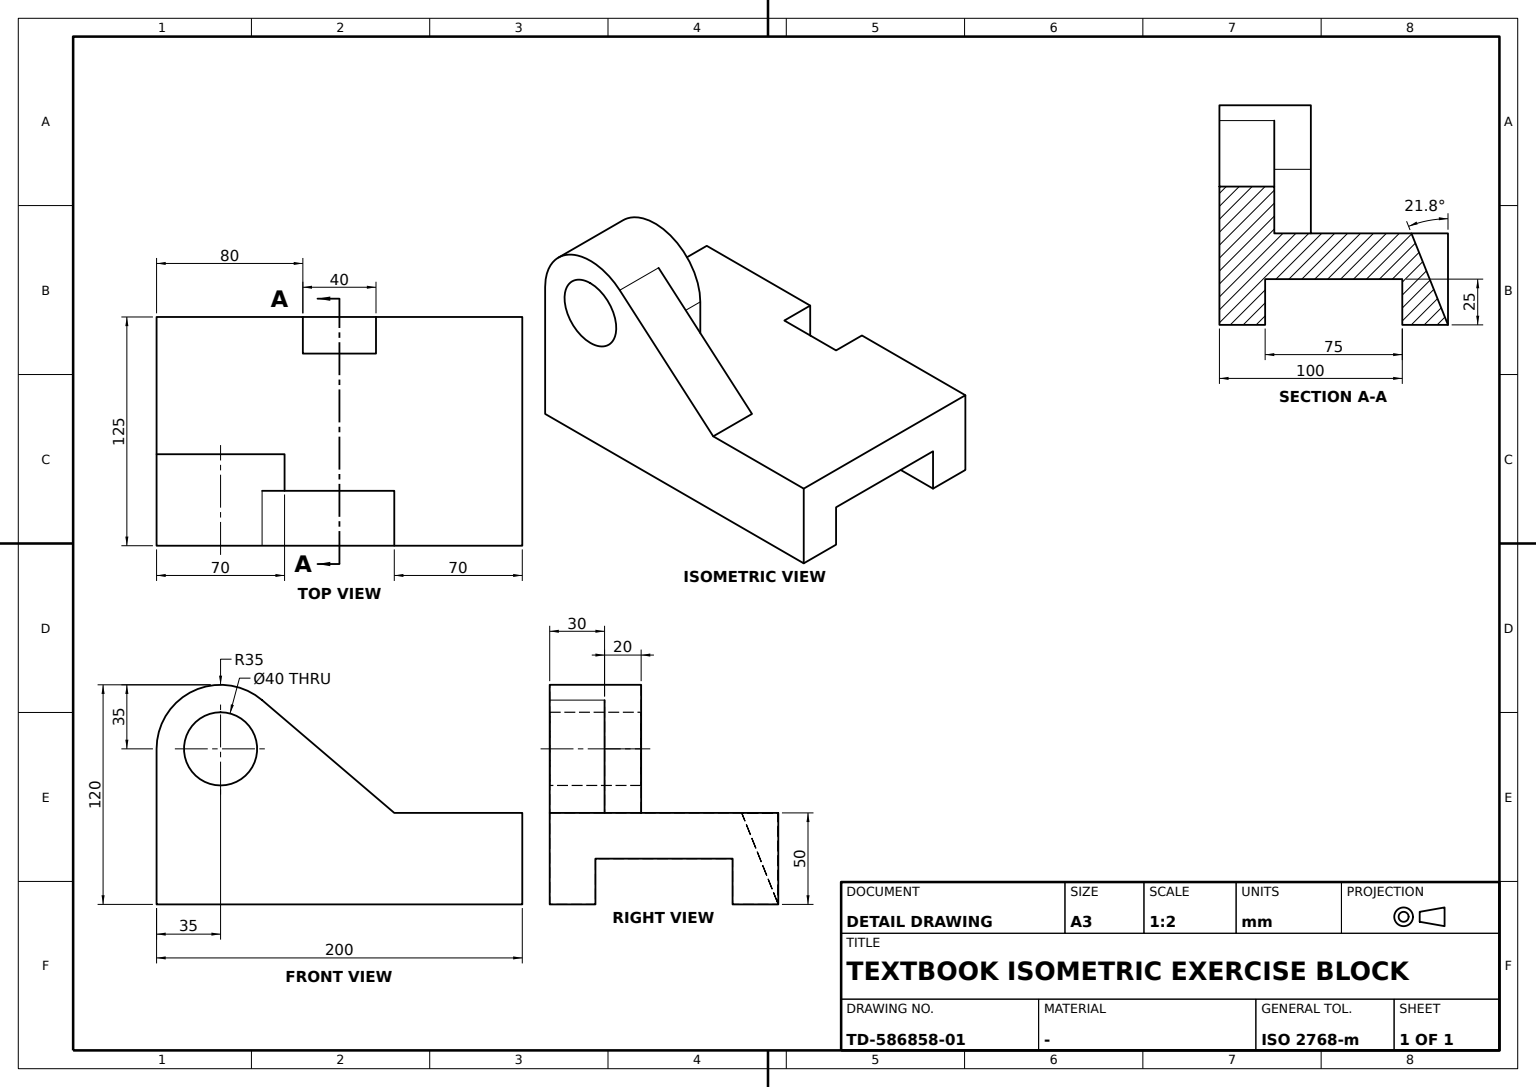
ISO-10303-21;
HEADER;
FILE_DESCRIPTION((''),'2;1');
FILE_NAME('','',(''),(''),'','','');
FILE_SCHEMA(('AUTOMOTIVE_DESIGN'));
ENDSEC;
DATA;
#1=APPLICATION_CONTEXT('');
#2=PRODUCT_CONTEXT('',#1,'mechanical');
#3=PRODUCT('','','',(#2));
#4=PRODUCT_DEFINITION_FORMATION('','',#3);
#5=PRODUCT_DEFINITION_CONTEXT('',#1,'design');
#6=PRODUCT_DEFINITION('','',#4,#5);
#7=PRODUCT_DEFINITION_SHAPE('','',#6);
#8=(LENGTH_UNIT()NAMED_UNIT(*)SI_UNIT(.MILLI.,.METRE.));
#9=(NAMED_UNIT(*)PLANE_ANGLE_UNIT()SI_UNIT($,.RADIAN.));
#10=(NAMED_UNIT(*)SI_UNIT($,.STERADIAN.)SOLID_ANGLE_UNIT());
#11=UNCERTAINTY_MEASURE_WITH_UNIT(LENGTH_MEASURE(0.005),#8,'distance_accuracy_value','');
#12=(GEOMETRIC_REPRESENTATION_CONTEXT(3)GLOBAL_UNCERTAINTY_ASSIGNED_CONTEXT((#11))GLOBAL_UNIT_ASSIGNED_CONTEXT((#8,#9,#10))REPRESENTATION_CONTEXT('',''));
#13=CARTESIAN_POINT('',(-20.,42.5,50.));
#14=VERTEX_POINT('',#13);
#15=CARTESIAN_POINT('',(-20.,62.5,0.));
#16=VERTEX_POINT('',#15);
#17=DIRECTION('',(0.,0.371390676,-0.928476691));
#18=VECTOR('',#17,1000.);
#19=LINE('',#13,#18);
#20=EDGE_CURVE('',#14,#16,#19,.T.);
#21=ORIENTED_EDGE('',*,*,#20,.T.);
#22=CARTESIAN_POINT('',(-20.,62.5,50.));
#23=VERTEX_POINT('',#22);
#24=DIRECTION('',(0.,0.,1.));
#25=VECTOR('',#24,1000.);
#26=LINE('',#22,#25);
#27=EDGE_CURVE('',#16,#23,#26,.T.);
#28=ORIENTED_EDGE('',*,*,#27,.T.);
#29=CARTESIAN_POINT('',(-20.,-62.5,50.));
#30=DIRECTION('',(0.,-1.,0.));
#31=VECTOR('',#30,1000.);
#32=LINE('',#29,#31);
#33=EDGE_CURVE('',#23,#14,#32,.T.);
#34=ORIENTED_EDGE('',*,*,#33,.T.);
#35=EDGE_LOOP('',(#21,#28,#34));
#36=FACE_BOUND('',#35,.T.);
#37=CARTESIAN_POINT('',(-20.,0.,0.));
#38=DIRECTION('',(1.,0.,0.));
#39=DIRECTION('',(0.,1.,0.));
#40=AXIS2_PLACEMENT_3D('',#37,#38,#39);
#41=PLANE('',#40);
#42=ADVANCED_FACE('',(#36),#41,.T.);
#43=CARTESIAN_POINT('',(-65.,-12.5,65.));
#44=VERTEX_POINT('',#43);
#45=CARTESIAN_POINT('',(-65.,-12.5,85.));
#46=DIRECTION('',(0.,0.,-1.));
#47=AXIS2_PLACEMENT_3D('',#45,#30,#46);
#48=CIRCLE('',#47,20.);
#49=EDGE_CURVE('',#44,#44,#48,.T.);
#50=ORIENTED_EDGE('',*,*,#49,.F.);
#51=EDGE_LOOP('',(#50));
#52=FACE_BOUND('',#51,.T.);
#53=CARTESIAN_POINT('',(-65.,-62.5,105.));
#54=VERTEX_POINT('',#53);
#55=CARTESIAN_POINT('',(-65.,-62.5,85.));
#56=AXIS2_PLACEMENT_3D('',#55,#39,#24);
#57=CIRCLE('',#56,20.);
#58=EDGE_CURVE('',#54,#54,#57,.F.);
#59=ORIENTED_EDGE('',*,*,#58,.T.);
#60=EDGE_LOOP('',(#59));
#61=FACE_BOUND('',#60,.T.);
#62=CARTESIAN_POINT('',(-65.,-37.5,85.));
#63=AXIS2_PLACEMENT_3D('',#62,#30,#38);
#64=CYLINDRICAL_SURFACE('',#63,20.);
#65=ADVANCED_FACE('',(#52,#61),#64,.F.);
#66=CARTESIAN_POINT('',(20.,62.5,50.));
#67=VERTEX_POINT('',#66);
#68=CARTESIAN_POINT('',(20.,42.5,50.));
#69=VERTEX_POINT('',#68);
#70=CARTESIAN_POINT('',(20.,-62.5,50.));
#71=LINE('',#70,#31);
#72=EDGE_CURVE('',#67,#69,#71,.T.);
#73=ORIENTED_EDGE('',*,*,#72,.F.);
#74=CARTESIAN_POINT('',(20.,62.5,0.));
#75=VERTEX_POINT('',#74);
#76=LINE('',#66,#25);
#77=EDGE_CURVE('',#75,#67,#76,.T.);
#78=ORIENTED_EDGE('',*,*,#77,.F.);
#79=LINE('',#68,#18);
#80=EDGE_CURVE('',#69,#75,#79,.T.);
#81=ORIENTED_EDGE('',*,*,#80,.F.);
#82=EDGE_LOOP('',(#73,#78,#81));
#83=FACE_BOUND('',#82,.T.);
#84=CARTESIAN_POINT('',(20.,0.,0.));
#85=AXIS2_PLACEMENT_3D('',#84,#38,#39);
#86=PLANE('',#85);
#87=ADVANCED_FACE('',(#83),#86,.F.);
#88=CARTESIAN_POINT('',(100.,-37.5,25.));
#89=VERTEX_POINT('',#88);
#90=CARTESIAN_POINT('',(100.,-37.5,0.));
#91=VERTEX_POINT('',#90);
#92=VECTOR('',#46,1000.);
#93=LINE('',#90,#92);
#94=EDGE_CURVE('',#89,#91,#93,.T.);
#95=ORIENTED_EDGE('',*,*,#94,.F.);
#96=CARTESIAN_POINT('',(100.,37.5,25.));
#97=VERTEX_POINT('',#96);
#98=CARTESIAN_POINT('',(100.,0.,25.));
#99=LINE('',#98,#31);
#100=EDGE_CURVE('',#97,#89,#99,.T.);
#101=ORIENTED_EDGE('',*,*,#100,.F.);
#102=CARTESIAN_POINT('',(100.,37.5,0.));
#103=VERTEX_POINT('',#102);
#104=LINE('',#102,#25);
#105=EDGE_CURVE('',#103,#97,#104,.T.);
#106=ORIENTED_EDGE('',*,*,#105,.F.);
#107=CARTESIAN_POINT('',(100.,62.5,0.));
#108=VERTEX_POINT('',#107);
#109=CARTESIAN_POINT('',(100.,0.,0.));
#110=LINE('',#109,#31);
#111=EDGE_CURVE('',#108,#103,#110,.T.);
#112=ORIENTED_EDGE('',*,*,#111,.F.);
#113=CARTESIAN_POINT('',(100.,62.5,50.));
#114=VERTEX_POINT('',#113);
#115=LINE('',#107,#92);
#116=EDGE_CURVE('',#114,#108,#115,.T.);
#117=ORIENTED_EDGE('',*,*,#116,.F.);
#118=CARTESIAN_POINT('',(100.,-62.5,50.));
#119=VERTEX_POINT('',#118);
#120=CARTESIAN_POINT('',(100.,0.,50.));
#121=VECTOR('',#39,1000.);
#122=LINE('',#120,#121);
#123=EDGE_CURVE('',#119,#114,#122,.T.);
#124=ORIENTED_EDGE('',*,*,#123,.F.);
#125=CARTESIAN_POINT('',(100.,-62.5,0.));
#126=VERTEX_POINT('',#125);
#127=LINE('',#125,#25);
#128=EDGE_CURVE('',#126,#119,#127,.T.);
#129=ORIENTED_EDGE('',*,*,#128,.F.);
#130=EDGE_CURVE('',#91,#126,#110,.T.);
#131=ORIENTED_EDGE('',*,*,#130,.F.);
#132=EDGE_LOOP('',(#95,#101,#106,#112,#117,#124,#129,#131));
#133=FACE_BOUND('',#132,.T.);
#134=AXIS2_PLACEMENT_3D('',#109,#38,#39);
#135=PLANE('',#134);
#136=ADVANCED_FACE('',(#133),#135,.T.);
#137=CARTESIAN_POINT('',(-100.,-12.5,50.));
#138=VERTEX_POINT('',#137);
#139=CARTESIAN_POINT('',(-30.,-12.5,50.));
#140=VERTEX_POINT('',#139);
#141=CARTESIAN_POINT('',(0.,-12.5,50.));
#142=VECTOR('',#38,1000.);
#143=LINE('',#141,#142);
#144=EDGE_CURVE('',#138,#140,#143,.T.);
#145=ORIENTED_EDGE('',*,*,#144,.F.);
#146=CARTESIAN_POINT('',(-100.,-12.5,85.));
#147=VERTEX_POINT('',#146);
#148=CARTESIAN_POINT('',(-100.,-12.5,0.));
#149=LINE('',#148,#92);
#150=EDGE_CURVE('',#147,#138,#149,.T.);
#151=ORIENTED_EDGE('',*,*,#150,.F.);
#152=CARTESIAN_POINT('',(-30.,-12.5,85.));
#153=VERTEX_POINT('',#152);
#154=CIRCLE('',#47,35.);
#155=EDGE_CURVE('',#153,#147,#154,.T.);
#156=ORIENTED_EDGE('',*,*,#155,.F.);
#157=LINE('',#139,#25);
#158=EDGE_CURVE('',#140,#153,#157,.T.);
#159=ORIENTED_EDGE('',*,*,#158,.F.);
#160=EDGE_LOOP('',(#145,#151,#156,#159));
#161=FACE_BOUND('',#160,.T.);
#162=ORIENTED_EDGE('',*,*,#49,.T.);
#163=EDGE_LOOP('',(#162));
#164=FACE_BOUND('',#163,.T.);
#165=CARTESIAN_POINT('',(0.,-12.5,0.));
#166=AXIS2_PLACEMENT_3D('',#165,#30,#38);
#167=PLANE('',#166);
#168=ADVANCED_FACE('',(#161,#164),#167,.F.);
#169=CARTESIAN_POINT('',(-100.,37.5,25.));
#170=VERTEX_POINT('',#169);
#171=CARTESIAN_POINT('',(0.,37.5,25.));
#172=LINE('',#171,#142);
#173=EDGE_CURVE('',#170,#97,#172,.T.);
#174=ORIENTED_EDGE('',*,*,#173,.T.);
#175=ORIENTED_EDGE('',*,*,#100,.T.);
#176=CARTESIAN_POINT('',(-100.,-37.5,25.));
#177=VERTEX_POINT('',#176);
#178=CARTESIAN_POINT('',(0.,-37.5,25.));
#179=LINE('',#178,#142);
#180=EDGE_CURVE('',#177,#89,#179,.T.);
#181=ORIENTED_EDGE('',*,*,#180,.F.);
#182=CARTESIAN_POINT('',(-100.,0.,25.));
#183=LINE('',#182,#31);
#184=EDGE_CURVE('',#170,#177,#183,.T.);
#185=ORIENTED_EDGE('',*,*,#184,.F.);
#186=EDGE_LOOP('',(#174,#175,#181,#185));
#187=FACE_BOUND('',#186,.T.);
#188=AXIS2_PLACEMENT_3D('',#171,#24,#30);
#189=PLANE('',#188);
#190=ADVANCED_FACE('',(#187),#189,.F.);
#191=CARTESIAN_POINT('',(-100.,62.5,50.));
#192=VERTEX_POINT('',#191);
#193=CARTESIAN_POINT('',(-100.,62.5,0.));
#194=VERTEX_POINT('',#193);
#195=LINE('',#193,#92);
#196=EDGE_CURVE('',#192,#194,#195,.T.);
#197=ORIENTED_EDGE('',*,*,#196,.F.);
#198=CARTESIAN_POINT('',(0.,62.5,50.));
#199=LINE('',#198,#142);
#200=EDGE_CURVE('',#192,#23,#199,.T.);
#201=ORIENTED_EDGE('',*,*,#200,.T.);
#202=ORIENTED_EDGE('',*,*,#27,.F.);
#203=CARTESIAN_POINT('',(0.,62.5,0.));
#204=LINE('',#203,#142);
#205=EDGE_CURVE('',#194,#16,#204,.T.);
#206=ORIENTED_EDGE('',*,*,#205,.F.);
#207=EDGE_LOOP('',(#197,#201,#202,#206));
#208=FACE_BOUND('',#207,.T.);
#209=AXIS2_PLACEMENT_3D('',#198,#30,#46);
#210=PLANE('',#209);
#211=ADVANCED_FACE('',(#208),#210,.F.);
#212=EDGE_CURVE('',#75,#108,#204,.T.);
#213=ORIENTED_EDGE('',*,*,#212,.T.);
#214=ORIENTED_EDGE('',*,*,#111,.T.);
#215=CARTESIAN_POINT('',(-100.,37.5,0.));
#216=VERTEX_POINT('',#215);
#217=CARTESIAN_POINT('',(0.,37.5,0.));
#218=LINE('',#217,#142);
#219=EDGE_CURVE('',#216,#103,#218,.T.);
#220=ORIENTED_EDGE('',*,*,#219,.F.);
#221=CARTESIAN_POINT('',(-100.,0.,0.));
#222=LINE('',#221,#31);
#223=EDGE_CURVE('',#194,#216,#222,.T.);
#224=ORIENTED_EDGE('',*,*,#223,.F.);
#225=ORIENTED_EDGE('',*,*,#205,.T.);
#226=DIRECTION('',(-1.,0.,0.));
#227=VECTOR('',#226,1000.);
#228=LINE('',#203,#227);
#229=EDGE_CURVE('',#75,#16,#228,.T.);
#230=ORIENTED_EDGE('',*,*,#229,.F.);
#231=EDGE_LOOP('',(#213,#214,#220,#224,#225,#230));
#232=FACE_BOUND('',#231,.T.);
#233=CARTESIAN_POINT('',(0.,-37.5,0.));
#234=AXIS2_PLACEMENT_3D('',#233,#24,#30);
#235=PLANE('',#234);
#236=ADVANCED_FACE('',(#232),#235,.F.);
#237=ORIENTED_EDGE('',*,*,#58,.F.);
#238=EDGE_LOOP('',(#237));
#239=FACE_BOUND('',#238,.T.);
#240=CARTESIAN_POINT('',(-42.292683,-62.5,111.634146));
#241=VERTEX_POINT('',#240);
#242=CARTESIAN_POINT('',(30.,-62.5,50.));
#243=VERTEX_POINT('',#242);
#244=CARTESIAN_POINT('',(37.31279,-62.5,43.765378));
#245=DIRECTION('',(0.76097561,0.,-0.648780488));
#246=VECTOR('',#245,1000.);
#247=LINE('',#244,#246);
#248=EDGE_CURVE('',#241,#243,#247,.T.);
#249=ORIENTED_EDGE('',*,*,#248,.F.);
#250=CARTESIAN_POINT('',(-100.,-62.5,85.));
#251=VERTEX_POINT('',#250);
#252=CIRCLE('',#56,35.);
#253=EDGE_CURVE('',#241,#251,#252,.F.);
#254=ORIENTED_EDGE('',*,*,#253,.T.);
#255=CARTESIAN_POINT('',(-100.,-62.5,0.));
#256=VERTEX_POINT('',#255);
#257=LINE('',#255,#25);
#258=EDGE_CURVE('',#256,#251,#257,.T.);
#259=ORIENTED_EDGE('',*,*,#258,.F.);
#260=CARTESIAN_POINT('',(0.,-62.5,0.));
#261=LINE('',#260,#142);
#262=EDGE_CURVE('',#256,#126,#261,.T.);
#263=ORIENTED_EDGE('',*,*,#262,.T.);
#264=ORIENTED_EDGE('',*,*,#128,.T.);
#265=CARTESIAN_POINT('',(0.,-62.5,50.));
#266=LINE('',#265,#142);
#267=EDGE_CURVE('',#243,#119,#266,.T.);
#268=ORIENTED_EDGE('',*,*,#267,.F.);
#269=EDGE_LOOP('',(#249,#254,#259,#263,#264,#268));
#270=FACE_BOUND('',#269,.T.);
#271=AXIS2_PLACEMENT_3D('',#260,#39,#24);
#272=PLANE('',#271);
#273=ADVANCED_FACE('',(#239,#270),#272,.F.);
#274=CARTESIAN_POINT('',(0.,42.5,50.));
#275=LINE('',#274,#227);
#276=EDGE_CURVE('',#69,#14,#275,.T.);
#277=ORIENTED_EDGE('',*,*,#276,.F.);
#278=ORIENTED_EDGE('',*,*,#80,.T.);
#279=ORIENTED_EDGE('',*,*,#229,.T.);
#280=ORIENTED_EDGE('',*,*,#20,.F.);
#281=EDGE_LOOP('',(#277,#278,#279,#280));
#282=FACE_BOUND('',#281,.T.);
#283=DIRECTION('',(0.,0.928476691,0.371390676));
#284=AXIS2_PLACEMENT_3D('',#274,#283,#17);
#285=PLANE('',#284);
#286=ADVANCED_FACE('',(#282),#285,.T.);
#287=CARTESIAN_POINT('',(-30.,-32.5,50.));
#288=VERTEX_POINT('',#287);
#289=CARTESIAN_POINT('',(-30.,-62.5,50.));
#290=LINE('',#289,#121);
#291=EDGE_CURVE('',#288,#140,#290,.T.);
#292=ORIENTED_EDGE('',*,*,#291,.T.);
#293=ORIENTED_EDGE('',*,*,#158,.T.);
#294=CARTESIAN_POINT('',(-30.,-32.5,85.));
#295=VERTEX_POINT('',#294);
#296=CARTESIAN_POINT('',(-30.,-37.5,85.));
#297=LINE('',#296,#31);
#298=EDGE_CURVE('',#295,#153,#297,.F.);
#299=ORIENTED_EDGE('',*,*,#298,.F.);
#300=LINE('',#287,#25);
#301=EDGE_CURVE('',#288,#295,#300,.T.);
#302=ORIENTED_EDGE('',*,*,#301,.F.);
#303=EDGE_LOOP('',(#292,#293,#299,#302));
#304=FACE_BOUND('',#303,.T.);
#305=AXIS2_PLACEMENT_3D('',#289,#226,#24);
#306=PLANE('',#305);
#307=ADVANCED_FACE('',(#304),#306,.F.);
#308=CARTESIAN_POINT('',(-100.,-37.5,0.));
#309=VERTEX_POINT('',#308);
#310=LINE('',#233,#142);
#311=EDGE_CURVE('',#309,#91,#310,.T.);
#312=ORIENTED_EDGE('',*,*,#311,.T.);
#313=ORIENTED_EDGE('',*,*,#130,.T.);
#314=ORIENTED_EDGE('',*,*,#262,.F.);
#315=EDGE_CURVE('',#309,#256,#222,.T.);
#316=ORIENTED_EDGE('',*,*,#315,.F.);
#317=EDGE_LOOP('',(#312,#313,#314,#316));
#318=FACE_BOUND('',#317,.T.);
#319=ADVANCED_FACE('',(#318),#235,.F.);
#320=CARTESIAN_POINT('',(-100.,-37.5,85.));
#321=LINE('',#320,#31);
#322=EDGE_CURVE('',#251,#147,#321,.F.);
#323=ORIENTED_EDGE('',*,*,#322,.F.);
#324=ORIENTED_EDGE('',*,*,#253,.F.);
#325=CARTESIAN_POINT('',(-42.292683,-32.5,111.634146));
#326=VERTEX_POINT('',#325);
#327=CARTESIAN_POINT('',(-42.292683,-37.5,111.634146));
#328=LINE('',#327,#31);
#329=EDGE_CURVE('',#241,#326,#328,.F.);
#330=ORIENTED_EDGE('',*,*,#329,.T.);
#331=CARTESIAN_POINT('',(-65.,-32.5,85.));
#332=AXIS2_PLACEMENT_3D('',#331,#30,#46);
#333=CIRCLE('',#332,35.);
#334=EDGE_CURVE('',#295,#326,#333,.T.);
#335=ORIENTED_EDGE('',*,*,#334,.F.);
#336=ORIENTED_EDGE('',*,*,#298,.T.);
#337=ORIENTED_EDGE('',*,*,#155,.T.);
#338=EDGE_LOOP('',(#323,#324,#330,#335,#336,#337));
#339=FACE_BOUND('',#338,.T.);
#340=CYLINDRICAL_SURFACE('',#63,35.);
#341=ADVANCED_FACE('',(#339),#340,.T.);
#342=ORIENTED_EDGE('',*,*,#267,.T.);
#343=ORIENTED_EDGE('',*,*,#123,.T.);
#344=EDGE_CURVE('',#67,#114,#199,.T.);
#345=ORIENTED_EDGE('',*,*,#344,.F.);
#346=ORIENTED_EDGE('',*,*,#72,.T.);
#347=ORIENTED_EDGE('',*,*,#276,.T.);
#348=ORIENTED_EDGE('',*,*,#33,.F.);
#349=ORIENTED_EDGE('',*,*,#200,.F.);
#350=CARTESIAN_POINT('',(-100.,0.,50.));
#351=LINE('',#350,#121);
#352=EDGE_CURVE('',#138,#192,#351,.T.);
#353=ORIENTED_EDGE('',*,*,#352,.F.);
#354=ORIENTED_EDGE('',*,*,#144,.T.);
#355=ORIENTED_EDGE('',*,*,#291,.F.);
#356=CARTESIAN_POINT('',(30.,-32.5,50.));
#357=VERTEX_POINT('',#356);
#358=CARTESIAN_POINT('',(0.,-32.5,50.));
#359=LINE('',#358,#142);
#360=EDGE_CURVE('',#288,#357,#359,.T.);
#361=ORIENTED_EDGE('',*,*,#360,.T.);
#362=LINE('',#242,#121);
#363=EDGE_CURVE('',#243,#357,#362,.T.);
#364=ORIENTED_EDGE('',*,*,#363,.F.);
#365=EDGE_LOOP('',(#342,#343,#345,#346,#347,#348,#349,#353,#354,#355,#361,#364));
#366=FACE_BOUND('',#365,.T.);
#367=AXIS2_PLACEMENT_3D('',#265,#46,#39);
#368=PLANE('',#367);
#369=ADVANCED_FACE('',(#366),#368,.F.);
#370=ORIENTED_EDGE('',*,*,#77,.T.);
#371=ORIENTED_EDGE('',*,*,#344,.T.);
#372=ORIENTED_EDGE('',*,*,#116,.T.);
#373=ORIENTED_EDGE('',*,*,#212,.F.);
#374=EDGE_LOOP('',(#370,#371,#372,#373));
#375=FACE_BOUND('',#374,.T.);
#376=ADVANCED_FACE('',(#375),#210,.F.);
#377=ORIENTED_EDGE('',*,*,#248,.T.);
#378=ORIENTED_EDGE('',*,*,#363,.T.);
#379=LINE('',#325,#246);
#380=EDGE_CURVE('',#326,#357,#379,.T.);
#381=ORIENTED_EDGE('',*,*,#380,.F.);
#382=ORIENTED_EDGE('',*,*,#329,.F.);
#383=EDGE_LOOP('',(#377,#378,#381,#382));
#384=FACE_BOUND('',#383,.T.);
#385=DIRECTION('',(0.648780488,0.,0.76097561));
#386=AXIS2_PLACEMENT_3D('',#240,#385,#245);
#387=PLANE('',#386);
#388=ADVANCED_FACE('',(#384),#387,.T.);
#389=ORIENTED_EDGE('',*,*,#150,.T.);
#390=ORIENTED_EDGE('',*,*,#352,.T.);
#391=ORIENTED_EDGE('',*,*,#196,.T.);
#392=ORIENTED_EDGE('',*,*,#223,.T.);
#393=LINE('',#215,#25);
#394=EDGE_CURVE('',#216,#170,#393,.T.);
#395=ORIENTED_EDGE('',*,*,#394,.T.);
#396=ORIENTED_EDGE('',*,*,#184,.T.);
#397=LINE('',#308,#92);
#398=EDGE_CURVE('',#177,#309,#397,.T.);
#399=ORIENTED_EDGE('',*,*,#398,.T.);
#400=ORIENTED_EDGE('',*,*,#315,.T.);
#401=ORIENTED_EDGE('',*,*,#258,.T.);
#402=ORIENTED_EDGE('',*,*,#322,.T.);
#403=EDGE_LOOP('',(#389,#390,#391,#392,#395,#396,#399,#400,#401,#402));
#404=FACE_BOUND('',#403,.T.);
#405=AXIS2_PLACEMENT_3D('',#221,#38,#39);
#406=PLANE('',#405);
#407=ADVANCED_FACE('',(#404),#406,.F.);
#408=ORIENTED_EDGE('',*,*,#105,.T.);
#409=ORIENTED_EDGE('',*,*,#173,.F.);
#410=ORIENTED_EDGE('',*,*,#394,.F.);
#411=ORIENTED_EDGE('',*,*,#219,.T.);
#412=EDGE_LOOP('',(#408,#409,#410,#411));
#413=FACE_BOUND('',#412,.T.);
#414=AXIS2_PLACEMENT_3D('',#217,#39,#24);
#415=PLANE('',#414);
#416=ADVANCED_FACE('',(#413),#415,.F.);
#417=ORIENTED_EDGE('',*,*,#398,.F.);
#418=ORIENTED_EDGE('',*,*,#180,.T.);
#419=ORIENTED_EDGE('',*,*,#94,.T.);
#420=ORIENTED_EDGE('',*,*,#311,.F.);
#421=EDGE_LOOP('',(#417,#418,#419,#420));
#422=FACE_BOUND('',#421,.T.);
#423=AXIS2_PLACEMENT_3D('',#178,#30,#46);
#424=PLANE('',#423);
#425=ADVANCED_FACE('',(#422),#424,.F.);
#426=ORIENTED_EDGE('',*,*,#360,.F.);
#427=ORIENTED_EDGE('',*,*,#301,.T.);
#428=ORIENTED_EDGE('',*,*,#334,.T.);
#429=ORIENTED_EDGE('',*,*,#380,.T.);
#430=EDGE_LOOP('',(#426,#427,#428,#429));
#431=FACE_BOUND('',#430,.T.);
#432=CARTESIAN_POINT('',(0.,-32.5,0.));
#433=AXIS2_PLACEMENT_3D('',#432,#30,#38);
#434=PLANE('',#433);
#435=ADVANCED_FACE('',(#431),#434,.F.);
#436=CLOSED_SHELL('',(#42,#65,#87,#136,#168,#190,#211,#236,#273,#286,#307,#319,#341,#369,#376,#388,#407,#416,#425,#435));
#437=MANIFOLD_SOLID_BREP('',#436);
#438=ADVANCED_BREP_SHAPE_REPRESENTATION('',(#437),#12);
#439=SHAPE_DEFINITION_REPRESENTATION(#7,#438);
ENDSEC;
END-ISO-10303-21;
